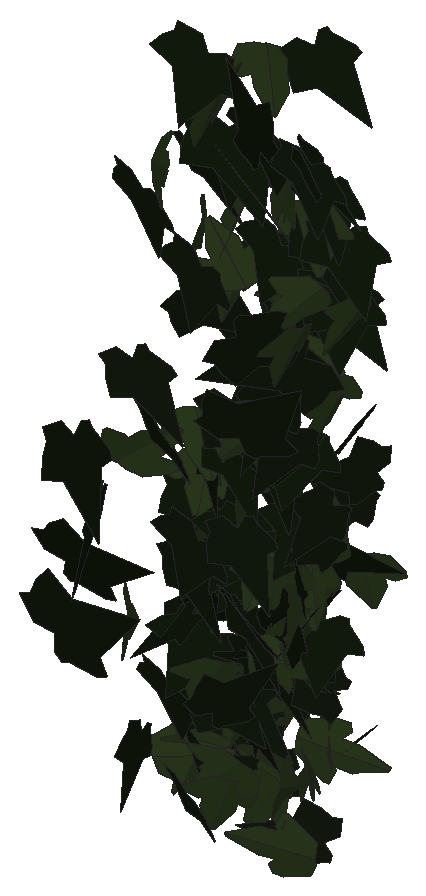
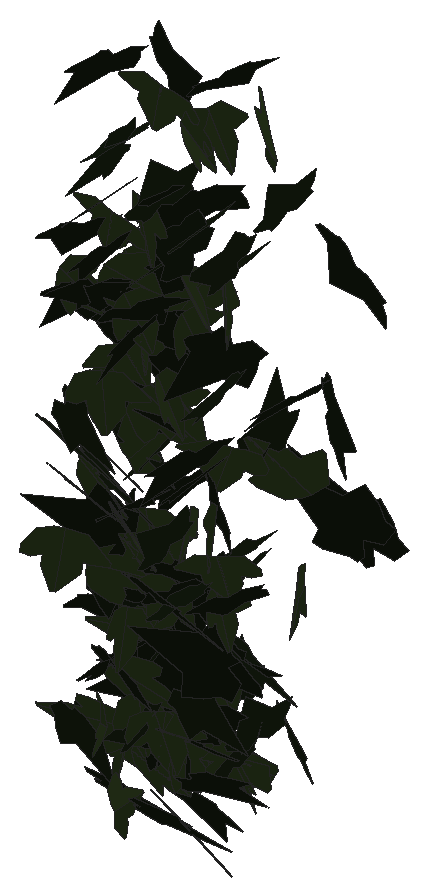
# SketchUp Ruby script. Lengths in inches.
U = 1.inch
M = Sketchup.active_model
def pt(a) = Geom::Point3d.new(a.map { |v| v * U })
def face(e, loops, mat)
  f = e.add_face(loops[0].map { |a| pt(a) })
  loops[1..].each { |l| e.add_face(l.map { |a| pt(a) }).erase! }
  f.material = f.back_material = mat if mat
  f
end
# faces: each face lists its corners as indices into pts; further lists are holes
def faces(e, pts, list, mat = nil) = list.each { |f| face(e, (f[0].is_a?(Array) ? f : [f]).map { |l| l.map { |i| pts[i] } }, mat) }
# xy, xz, yz: faces in a plane at the given z, y or x. An outline is a flat list of corners, or four numbers for a rectangle; further outlines are holes
def ring(l) = l.size == 4 ? [[l[0], l[1]], [l[2], l[1]], [l[2], l[3]], [l[0], l[3]]] : l.each_slice(2).to_a
def flat(e, list, mat, &to3) = list.each { |f| face(e, (f[0].is_a?(Array) ? f : [f]).map { |l| ring(l).map { |u, v| to3.(u, v) } }, mat) }
def xy(e, z, list, mat = nil) = flat(e, list, mat) { |x, y| [x, y, z] }
def xz(e, y, list, mat = nil) = flat(e, list, mat) { |x, z| [x, y, z] }
def yz(e, x, list, mat = nil) = flat(e, list, mat) { |y, z| [x, y, z] }
def lines(e, pts, list) = list.each { |a, b| e.add_line(pt(pts[a]), pt(pts[b])) }
# prism: a flat outline (further loops are holes) pulled along v
def prism(e, loops, v, mat = nil)
  f = face(e, loops, mat); d = Geom::Vector3d.new(v.map { |x| x * U })
  f.pushpull(f.normal.samedirection?(d) ? d.length : -d.length)
end
def box(e, o, s, mat = nil) = prism(e, [[o, [o[0] + s[0], o[1], o[2]], [o[0] + s[0], o[1] + s[1], o[2]], [o[0], o[1] + s[1], o[2]]]], [0, 0, s[2]], mat)
def at(x, y, z, deg = 0) = Geom::Transformation.translation(pt([x, y, z])) * Geom::Transformation.rotation(ORIGIN, Z_AXIS, deg.degrees)
def axes(o, x, y, z) = Geom::Transformation.new([*x, 0, *y, 0, *z, 0, *pt(o).to_a, 1])
def part(name) = M.definitions.add(name)
# library, detail: a bought-in or finely detailed component or shape, given as its bounding box
def library(name, o, s) = part(name).tap { |d| box(d.entities, o, s) }
def detail(e, o, s) = box(e.add_group.entities, o, s)
def put(e, d, t, mat = nil) = e.add_instance(d, t).tap { |i| i.material = mat if mat }
def group(e, t, mat = nil) = e.add_group.tap { |g| g.transformation = t; g.material = mat if mat }.entities
root = M.entities
M.materials.add("1026 AP 7946 SUNNY SIDE UP").color = [254, 231, 186]
M.materials.add("efeu1").color = [18, 25, 13]
M.materials.add("efeu2").color = [43, 57, 29]
c1 = part("ivyleaf_9")
p = [[1.54,2.16,1.25],[1.36,2.04,1.19],[-0.21,0.99,0.68],[-0.71,1.11,0.82],[-0.85,0.86,0.67],[-0.8,0.17,0.21],
  [-0.9,-0.01,0.1],[-0.67,-0.16,-0.02],[-0.08,-0.08,-0.05],[-0.03,-0.6,-0.4],[0.65,-0.88,-0.66],[0.83,-0.6,-0.49],
  [1.29,-0.42,-0.43],[1.8125,-0.07,-0.26],[1.21,0.44,0.15]]
faces(c1.entities,p,[[0,1,2,3,4,5,6,7,8,9,10,11,12,13,14]],"efeu1")
c2 = part("ivyleaf_10")
p = [[0,0.5,-0.03],[-0.0625,2.02,-0.43],[-0.19,2.01,-0.46],[-0.54,1.05,-0.29],[-0.52,0.625,-0.18],[-0.83,0.76,-0.28],
  [-1.16,0.64,-0.33],[-1.15,0.33,-0.24],[-0.77,-0.39,0.02],[-0.3,-0.51,0.16],[0.04,-0.48,0.23],[-0.02,2.01,-0.4375],
  [-0.06,2.01,-0.43],[0.04,-0.49,0.23],[0.67,-0.49,0.14],[1.38,0.36,-0.2],[1.375,0.51,-0.24],[0.81,0.65,-0.19],
  [0.62,0.59,-0.15],[0.6,1.09,-0.28],[0.5,1.23,-0.31]]
faces(c2.entities,p,[[0,1,2,3,4,5,6,7,8,9,10],[11,12,0,13,14,15,16,17,18,19,20]],"efeu2")
put(root,c1,axes([128.98,212.18,288.85],[0.31029,-0.29326,0.02774],[0.02209,-0.02501,-0.36428],[0.46278,0.19782,-0.00121]),"1026 AP 7946 SUNNY SIDE UP")
put(root,c2,axes([129.09,210.67,284.76],[-0.31965,-0.18826,0.23279],[0.23188,0.17392,0.28561],[-0.40163,0.25025,-0.02038]),"1026 AP 7946 SUNNY SIDE UP")
put(root,c1,axes([129.04,210.82,286.14],[0.1394,-0.3386,-0.12751],[0.0207,0.12846,-0.35713],[0.56545,0.07877,0.04451]),"1026 AP 7946 SUNNY SIDE UP")
put(root,c1,axes([129.14,212.12,283.58],[-0.05305,-0.33119,-0.07714],[0.03232,0.07122,-0.34228],[0.53228,-0.03734,0.0131]),"1026 AP 7946 SUNNY SIDE UP")
put(root,c2,axes([129.27,212.125,284.0625],[0.45145,0.17881,-0.05168],[-0.04942,-0.04614,-0.34796],[-0.28825,0.28796,-0.02128]),"1026 AP 7946 SUNNY SIDE UP")
put(root,c1,axes([128.88,209.61,283.53],[0.07526,-0.04022,0.3979],[0.48083,-0.23633,-0.06574],[0.37693,0.3095,0.00441]),"1026 AP 7946 SUNNY SIDE UP")
put(root,c2,axes([129.44,211.78,288.09],[0.15161,-0.31162,-0.1802],[-0.01395,0.17722,-0.33263],[0.56039,0.08872,0.04047]),"1026 AP 7946 SUNNY SIDE UP")
put(root,c1,axes([129.16,212.22,286.77],[0.23192,-0.3104,-0.0389],[-0.03271,0.02997,-0.35381],[0.49025,0.14884,-0.0052]),"1026 AP 7946 SUNNY SIDE UP")
put(root,c1,axes([129.63,211.27,282.24],[-0.41649,0.14606,-0.1242],[0.11868,-0.1102,-0.30691],[-0.27403,-0.26972,0.05584]),"1026 AP 7946 SUNNY SIDE UP")
put(root,c2,axes([129.53,211.8,283.26],[-0.04126,-0.32542,-0.02046],[-0.0011,0.01813,-0.33622],[0.51247,-0.02616,-0.00237]),"1026 AP 7946 SUNNY SIDE UP")
put(root,c2,axes([129.63,211.86,284.52],[-0.14659,0.22989,0.23773],[-0.24344,0.17841,-0.2479],[-0.44899,-0.17179,0.05679]),"1026 AP 7946 SUNNY SIDE UP")
put(root,c1,axes([129.25,210.73,288.93],[0.05276,-0.30959,0.21871],[0.07883,-0.20932,-0.32119],[0.58655,0.05598,0.02349]),"1026 AP 7946 SUNNY SIDE UP")
put(root,c2,axes([129.57,210,282.73],[0.14073,-0.21398,-0.33372],[-0.02347,0.32908,-0.22712],[0.60841,0.06219,0.06843]),"1026 AP 7946 SUNNY SIDE UP")
put(root,c1,axes([129.75,212.03,280.51],[-0.44826,-0.1148,0.09985],[-0.12089,-0.06874,-0.31513],[0.20373,-0.29337,0.0327]),"1026 AP 7946 SUNNY SIDE UP")
put(root,c1,axes([129.45,210.42,280.66],[-0.29729,0.01639,-0.31],[0.43122,-0.13818,-0.18602],[-0.19681,-0.32751,0.0607]),"1026 AP 7946 SUNNY SIDE UP")
put(root,c1,axes([129.34,211.22,281],[-0.02633,-0.26581,0.24746],[0.1188,-0.23918,-0.26696],[0.5523,0.03878,0.06922]),"1026 AP 7946 SUNNY SIDE UP")
put(root,c1,axes([129.56,211.5625,287.07],[-0.00988,-0.08955,-0.36536],[-0.03579,0.3536,-0.08963],[0.57326,0.02053,-0.01189]),"1026 AP 7946 SUNNY SIDE UP")
put(root,c1,axes([129.48,210.8,285.26],[0.40755,-0.2427,-0.19779],[0.25328,-0.10593,0.36397],[-0.4139,-0.3038,0.02797]),"1026 AP 7946 SUNNY SIDE UP")
put(root,c1,axes([129.57,212.22,289.14],[-0.01928,-0.32385,0.14098],[0.0022,-0.13882,-0.33462],[0.55394,-0.01072,0.00623]),"1026 AP 7946 SUNNY SIDE UP")
put(root,c1,axes([129.31,208.84,282.92],[-0.04634,0.08615,0.46305],[0.4592,-0.34261,0.08547],[0.55308,0.29167,-0.03217]),"1026 AP 7946 SUNNY SIDE UP")
put(root,c1,axes([129.93,211.96,281.73],[-0.25677,0.20577,-0.20613],[0.09457,-0.20189,-0.2641],[-0.44259,-0.16252,0.06316]),"1026 AP 7946 SUNNY SIDE UP")
put(root,c2,axes([129.77,212.13,288.15],[0.27324,-0.30063,0.10989],[0.05657,-0.10417,-0.35774],[0.4993,0.17632,-0.0196]),"1026 AP 7946 SUNNY SIDE UP")
put(root,c1,axes([129.59,211.45,280.53],[0.01277,-0.26341,0.28842],[0.03471,-0.28075,-0.27297],[0.60516,0.02166,0.00957]),"1026 AP 7946 SUNNY SIDE UP")
put(root,c1,axes([129.6,211.74,284.6875],[-0.15114,-0.00468,-0.3375],[0.49212,-0.10221,-0.0937],[-0.15225,-0.32573,0.03216]),"1026 AP 7946 SUNNY SIDE UP")
put(root,c1,axes([129.89,211.37,281.95],[-0.42373,-0.2031,-0.00622],[0.02623,-0.01404,-0.34702],[0.31836,-0.26916,0.02032]),"1026 AP 7946 SUNNY SIDE UP")
put(root,c1,axes([129.74,209.17,284.96],[-0.30278,0.08323,-0.42338],[0.5409,-0.22815,-0.21473],[-0.3783,-0.39283,0.03184]),"1026 AP 7946 SUNNY SIDE UP")
put(root,c2,axes([129.89,211,280.27],[0.32015,-0.2617,-0.01845],[-0.03294,0.00449,-0.34127],[0.41099,0.20422,-0.01298]),"1026 AP 7946 SUNNY SIDE UP")
put(root,c1,axes([130.23,211.95,279.81],[-0.2866,0.22726,0.15585],[-0.16229,0.10936,-0.29927],[-0.3962,-0.20919,0.00986]),"1026 AP 7946 SUNNY SIDE UP")
put(root,c2,axes([129.9,211.96,290.4375],[0.15864,-0.30207,0.16275],[0.04643,-0.15818,-0.32838],[0.53525,0.10325,-0.01975]),"1026 AP 7946 SUNNY SIDE UP")
put(root,c1,axes([129.57,211.67,282.18],[0.24071,0.27262,-0.17899],[0.09189,0.16746,0.32187],[0.50129,-0.16161,0.02694]),"1026 AP 7946 SUNNY SIDE UP")
put(root,c2,axes([129.97,211.35,290.31],[-0.01407,-0.35184,0.06304],[0.00713,-0.06332,-0.3629],[0.56205,-0.00801,0.00618]),"1026 AP 7946 SUNNY SIDE UP")
put(root,c2,axes([129.74,211.32,285.24],[0.474,0.18788,0.07671],[0.12034,0.01557,-0.3648],[-0.29344,0.30986,-0.0257]),"1026 AP 7946 SUNNY SIDE UP")
put(root,c2,axes([129.78,211.0625,280.4],[-0.36542,-0.13235,-0.18939],[0.27678,0.05857,-0.27345],[0.22267,-0.29,0.02909]),"1026 AP 7946 SUNNY SIDE UP")
put(root,c1,axes([129.78,212.4,283.36],[-0.07065,-0.29446,0.19494],[0.05816,-0.19536,-0.30261],[0.54872,-0.01721,0.05718]),"1026 AP 7946 SUNNY SIDE UP")
put(root,c1,axes([129.91,211.3,291],[-0.21379,-0.33817,0.12317],[-0.04298,-0.11978,-0.37571],[0.56338,-0.13747,0.01808]),"1026 AP 7946 SUNNY SIDE UP")
put(root,c1,axes([129.73,211.01,283.26],[0.20783,-0.33524,-0.04471],[-0.04431,0.03347,-0.37076],[0.5293,0.13444,-0.01348]),"1026 AP 7946 SUNNY SIDE UP")
put(root,c2,axes([129.6,210.89,280.2],[0.19503,-0.05407,-0.30723],[0.46486,0.09119,0.11028],[0.10288,-0.30956,0.08413]),"1026 AP 7946 SUNNY SIDE UP")
put(root,c2,axes([129.74,210.48,289.64],[0.08213,-0.17038,-0.37165],[0.19188,-0.33856,0.18143],[-0.59583,-0.13251,0.0072]),"1026 AP 7946 SUNNY SIDE UP")
put(root,c1,axes([129.86,211.16,283.5],[-0.14287,-0.28812,0.20162],[0.01636,-0.20606,-0.3062],[0.54888,-0.06886,0.06161]),"1026 AP 7946 SUNNY SIDE UP")
put(root,c2,axes([129.98,211.9,287.41],[-0.07131,-0.31594,0.14114],[0.07394,-0.14434,-0.3235],[0.53755,-0.02206,0.06322]),"1026 AP 7946 SUNNY SIDE UP")
put(root,c1,axes([129.83,211.93,289.51],[-0.13347,-0.34189,-0.20315],[0.09331,0.18635,-0.36164],[0.61201,-0.10297,0.01083]),"1026 AP 7946 SUNNY SIDE UP")
put(root,c1,axes([130.09,211.68,279.98],[-0.45971,-0.04195,-0.13367],[0.20684,-0.00801,-0.30328],[0.05515,-0.31966,0.02323]),"1026 AP 7946 SUNNY SIDE UP")
put(root,c2,axes([130.16,211.625,287.58],[0.20429,0.34869,0.07074],[-0.08425,-0.05094,0.38163],[0.55182,-0.13687,0.03208]),"1026 AP 7946 SUNNY SIDE UP")
put(root,c2,axes([130.07,211.93,280.66],[-0.06327,-0.26305,0.17177],[0.06523,-0.17262,-0.26886],[0.48662,-0.01106,0.05837]),"1026 AP 7946 SUNNY SIDE UP")
put(root,c1,axes([129.74,212.18,288.74],[0.25367,-0.2557,0.21436],[0.16216,-0.18259,-0.31242],[0.49387,0.19129,-0.00752]),"1026 AP 7946 SUNNY SIDE UP")
put(root,c1,axes([129.98,211.07,287.83],[-0.07442,-0.31588,0.19649],[0.0005,-0.19413,-0.32918],[0.58167,-0.04025,0.02542]),"1026 AP 7946 SUNNY SIDE UP")
put(root,c1,axes([130.44,211.88,280.92],[-0.4647,0.03392,0.10972],[-0.17546,-0.09083,-0.29026],[0.00058,-0.30065,0.09812]),"1026 AP 7946 SUNNY SIDE UP")
put(root,c2,axes([130.26,211.1,281.66],[-0.27905,-0.2664,0.10917],[-0.07268,-0.09821,-0.32997],[0.44581,-0.18276,0.01454]),"1026 AP 7946 SUNNY SIDE UP")
put(root,c2,axes([130.35,212.12,281.19],[-0.42749,-0.14965,0.09816],[-0.11783,-0.06288,-0.31953],[0.25364,-0.28143,0.01701]),"1026 AP 7946 SUNNY SIDE UP")
put(root,c1,axes([129.97,211.82,285.37],[0.11708,-0.3568,-0.21301],[-0.03229,0.20459,-0.37379],[0.64603,0.07489,0.01992]),"1026 AP 7946 SUNNY SIDE UP")
put(root,c2,axes([130.25,212.08,286.4],[0.08507,-0.34302,0.04229],[0.0026,-0.04327,-0.35796],[0.54358,0.05389,-0.00491]),"1026 AP 7946 SUNNY SIDE UP")
put(root,c2,axes([130.21,211.57,284.16],[0.21798,-0.21477,-0.21885],[0.04701,0.24117,-0.23101],[0.47131,0.07528,0.12426]),"1026 AP 7946 SUNNY SIDE UP")
put(root,c2,axes([130.33,211.98,280.93],[-0.07069,0.29943,-0.20892],[-0.03244,0.20361,0.313],[0.56922,0.04879,-0.00811]),"1026 AP 7946 SUNNY SIDE UP")
put(root,c1,axes([130.33,211.79,283.52],[-0.43734,-0.19791,-0.00507],[0.02987,-0.02017,-0.35065],[0.30982,-0.27743,0.02665]),"1026 AP 7946 SUNNY SIDE UP")
put(root,c1,axes([130.59,212.15,283.27],[-0.53377,0.11963,0.02066],[-0.04705,-0.02689,-0.36916],[-0.18466,-0.33895,0.03434]),"1026 AP 7946 SUNNY SIDE UP")
put(root,c1,axes([130.32,211.85,283.16],[-0.28947,-0.2616,0.07292],[-0.05448,-0.06395,-0.32981],[0.42326,-0.18714,0.00742]),"1026 AP 7946 SUNNY SIDE UP")
put(root,c1,axes([130.65,212.01,279.74],[-0.43261,0.08348,0.13003],[-0.21368,-0.02327,-0.29054],[-0.10325,-0.3016,0.0565]),"1026 AP 7946 SUNNY SIDE UP")
put(root,c1,axes([130.1,211.6,284.86],[0.08809,-0.35626,-0.02097],[-0.0143,0.01713,-0.37137],[0.56074,0.05641,-0.00618]),"1026 AP 7946 SUNNY SIDE UP")
put(root,c1,axes([130.03,212.29,284.18],[0.15924,-0.30773,0.14662],[0.07574,-0.13581,-0.33453],[0.52888,0.11211,0.00376]),"1026 AP 7946 SUNNY SIDE UP")
put(root,c1,axes([130.27,211.86,281],[-0.13516,-0.28439,-0.17093],[0.08103,0.15605,-0.30513],[0.51004,-0.10016,0.00318]),"1026 AP 7946 SUNNY SIDE UP")
put(root,c1,axes([130.17,212.26,289.41],[-0.03595,-0.30299,0.27858],[0.12253,-0.27078,-0.30543],[0.62855,0.03546,0.07548]),"1026 AP 7946 SUNNY SIDE UP")
put(root,c1,axes([130.19,211.33,281.2],[-0.0263,-0.18766,-0.30519],[0.26953,0.2532,-0.17436],[0.47942,-0.15264,0.08128]),"1026 AP 7946 SUNNY SIDE UP")
put(root,c1,axes([130.15,211.41,282.52],[0.25666,-0.18081,0.22477],[0.18419,-0.18751,-0.25029],[0.40708,0.19884,-0.02847]),"1026 AP 7946 SUNNY SIDE UP")
put(root,c1,axes([130.21,208.06,286.55],[-0.27026,-0.07851,-0.42642],[0.66177,-0.03067,-0.17441],[0.00206,-0.44673,0.08421]),"1026 AP 7946 SUNNY SIDE UP")
put(root,c2,axes([130.5,211.66,282.97],[-0.47387,0.10493,-0.0785],[0.10243,-0.04593,-0.32828],[-0.17695,-0.30759,0.0202]),"1026 AP 7946 SUNNY SIDE UP")
put(root,c1,axes([130.22,211.74,280.77],[0.1249,-0.0816,-0.36921],[0.55808,-0.0765,0.09866],[-0.1475,-0.35856,0.06067]),"1026 AP 7946 SUNNY SIDE UP")
put(root,c1,axes([130.59,212.34,287.66],[-0.27499,-0.30562,0.06225],[-0.02113,-0.06382,-0.36255],[0.48994,-0.17429,0.0193]),"1026 AP 7946 SUNNY SIDE UP")
put(root,c2,axes([130.42,211.94,290.86],[0.54317,-0.00947,0.1118],[0.17042,-0.00835,-0.35601],[0.01813,0.36201,-0.00317]),"1026 AP 7946 SUNNY SIDE UP")
put(root,c2,axes([130.875,210.65,280.55],[-0.41934,-0.04506,0.1981],[-0.27105,-0.10543,-0.272],[0.15237,-0.31158,0.06132]),"1026 AP 7946 SUNNY SIDE UP")
put(root,c2,axes([131.03,211.51,280.16],[0.03821,-0.06202,-0.35009],[-0.42407,0.20891,-0.05798],[0.33854,0.26869,-0.03312]),"1026 AP 7946 SUNNY SIDE UP")
put(root,c2,axes([131.02,211.95,281.68],[0.20781,-0.02697,-0.31376],[-0.46841,0.06264,-0.13859],[0.10723,0.32589,0.00267]),"1026 AP 7946 SUNNY SIDE UP")
put(root,c2,axes([130.93,211.43,285.66],[-0.27437,-0.2565,0.2591],[-0.19265,-0.22207,-0.32034],[0.53271,-0.21242,0.0176]),"1026 AP 7946 SUNNY SIDE UP")
put(root,c2,axes([130.82,210.64,280.21],[-0.34326,-0.23742,0.07887],[-0.05126,-0.07551,-0.3316],[0.38955,-0.21915,0.02587]),"1026 AP 7946 SUNNY SIDE UP")
put(root,c2,axes([130.74,211.93,288.94],[0.38784,-0.22497,-0.11929],[-0.04237,0.13573,-0.33369],[0.39466,0.23565,0.0814]),"1026 AP 7946 SUNNY SIDE UP")
put(root,c1,axes([130.64,211.97,288],[-0.12196,-0.29183,0.19282],[-0.02555,-0.19021,-0.31084],[0.54595,-0.07409,0.02852]),"1026 AP 7946 SUNNY SIDE UP")
put(root,c1,axes([130.41,211.36,281.86],[0.1263,0.00693,-0.32666],[0.27861,0.27036,0.0539],[0.4137,-0.18419,0.06343]),"1026 AP 7946 SUNNY SIDE UP")
put(root,c2,axes([130.84,211.88,281.1875],[-0.25378,-0.28316,0.00827],[0.01653,-0.01707,-0.33538],[0.44519,-0.16078,0.01717]),"1026 AP 7946 SUNNY SIDE UP")
put(root,c1,axes([130.55,212.14,281.18],[0.27127,-0.28105,0.01707],[-0.00698,-0.02401,-0.33946],[0.44279,0.1718,-0.01581]),"1026 AP 7946 SUNNY SIDE UP")
put(root,c1,axes([130.46,211.5,281.57],[0.37132,0.08955,0.22023],[0.33491,0.03466,-0.25776],[-0.14183,0.3163,-0.03209]),"1026 AP 7946 SUNNY SIDE UP")
put(root,c2,axes([130.87,212.03,287.43],[-0.13479,-0.32378,0.11475],[0.01275,-0.11859,-0.34373],[0.5392,-0.07814,0.03682]),"1026 AP 7946 SUNNY SIDE UP")
put(root,c1,axes([130.59,211.34,282.55],[0.17324,-0.33325,0.0462],[0.00667,-0.0478,-0.36169],[0.52909,0.10972,-0.01057]),"1026 AP 7946 SUNNY SIDE UP")
put(root,c1,axes([130.7,212.07,287.16],[0.19216,-0.28818,-0.19931],[-0.13759,0.17112,-0.32124],[0.52667,0.14985,-0.0112]),"1026 AP 7946 SUNNY SIDE UP")
put(root,c2,axes([130.875,212.33,279.83],[-0.11175,0.05265,-0.32907],[-0.06392,-0.32619,-0.04793],[-0.50548,0.02961,0.07881]),"1026 AP 7946 SUNNY SIDE UP")
put(root,c2,axes([130.92,212.0625,282.58],[-0.09734,-0.30946,-0.12062],[0.08296,0.10656,-0.32312],[0.51261,-0.07601,0.02939]),"1026 AP 7946 SUNNY SIDE UP")
put(root,c2,axes([130.92,211.3125,283.51],[0.29384,0.25441,-0.14933],[-0.10083,-0.13398,-0.32495],[-0.45039,0.19597,-0.02468]),"1026 AP 7946 SUNNY SIDE UP")
put(root,c2,axes([131.09,211.66,284.99],[-0.13959,-0.11042,-0.344],[-0.20257,-0.30956,0.1392],[-0.51357,0.15211,0.0386]),"1026 AP 7946 SUNNY SIDE UP")
put(root,c1,axes([131.27,210.72,290.32],[0.00792,-0.00458,0.42375],[-0.16731,0.39738,0.00822],[-0.62485,-0.10646,0.00317]),"1026 AP 7946 SUNNY SIDE UP")
put(root,c1,axes([130.78,209.8,280.47],[0.34127,-0.18212,-0.18513],[0.23814,-0.09681,0.29061],[-0.32283,-0.26393,0.01866]),"1026 AP 7946 SUNNY SIDE UP")
put(root,c2,axes([131.13,211.56,287.06],[0.12315,-0.32267,-0.18992],[-0.06581,0.17766,-0.34102],[0.57918,0.08879,0.00163]),"1026 AP 7946 SUNNY SIDE UP")
put(root,c2,axes([130.8,211.86,283.52],[0.29843,-0.22859,-0.18702],[0.25267,-0.09714,0.30067],[-0.38166,-0.24304,0.05282]),"1026 AP 7946 SUNNY SIDE UP")
put(root,c1,axes([130.92,210.73,284.2],[0.06829,-0.34078,-0.123],[-0.046,0.11459,-0.35296],[0.56491,0.05052,-0.01387]),"1026 AP 7946 SUNNY SIDE UP")
put(root,c1,axes([130.91,211.54,284.91],[0.07036,-0.31204,0.11333],[0.00694,-0.11222,-0.32521],[0.52113,0.04362,-0.01097]),"1026 AP 7946 SUNNY SIDE UP")
put(root,c2,axes([131.12,211.87,286.63],[0.34976,0.24975,-0.14014],[-0.13255,-0.10892,-0.34506],[-0.42821,0.23771,-0.00765]),"1026 AP 7946 SUNNY SIDE UP")
put(root,c1,axes([130.88,211.35,281.99],[0.31958,-0.29615,-0.06152],[-0.07751,0.03645,-0.36926],[0.46815,0.2082,-0.01914]),"1026 AP 7946 SUNNY SIDE UP")
put(root,c1,axes([131.18,211.31,286.18],[-0.52141,0.05376,-0.24378],[0.35468,-0.08085,-0.34458],[-0.14196,-0.39945,0.03446]),"1026 AP 7946 SUNNY SIDE UP")
put(root,c1,axes([131.55,211.3,286.86],[0.00731,-0.04482,-0.41684],[-0.38535,-0.3231,0.0321],[-0.51064,0.24319,-0.03019]),"1026 AP 7946 SUNNY SIDE UP")
put(root,c1,axes([130.98,210.69,287.26],[0.04697,0.02241,-0.41924],[-0.0406,0.40745,0.02354],[0.63977,0.02421,0.03227]),"1026 AP 7946 SUNNY SIDE UP")
put(root,c2,axes([131.31,211.15,283.58],[-0.43655,-0.17235,0.06034],[-0.05159,-0.05949,-0.33531],[0.28205,-0.27765,0.03206]),"1026 AP 7946 SUNNY SIDE UP")
put(root,c1,axes([131.125,212.05,281.78],[-0.35791,-0.01626,-0.24221],[0.36982,-0.03437,-0.23242],[-0.02119,-0.32536,0.03473]),"1026 AP 7946 SUNNY SIDE UP")
put(root,c2,axes([131.42,211.89,283.13],[-0.08203,-0.10298,0.36152],[-0.19561,-0.32897,-0.12023],[0.54171,-0.13438,0.01133]),"1026 AP 7946 SUNNY SIDE UP")
put(root,c2,axes([131.34,212.09,286.1],[-0.4154,-0.20689,0.02255],[-0.00541,-0.03292,-0.34501],[0.32729,-0.26313,0.02292]),"1026 AP 7946 SUNNY SIDE UP")
put(root,c2,axes([131.32,211.72,280.36],[-0.27957,0.24998,0.07178],[-0.10418,0.03618,-0.31406],[-0.39391,-0.18698,0.03211]),"1026 AP 7946 SUNNY SIDE UP")
put(root,c1,axes([131.61,211,283],[0.05018,-0.00341,-0.39736],[-0.60213,0.04602,-0.03279],[0.07256,0.38426,0.00269]),"1026 AP 7946 SUNNY SIDE UP")
put(root,c2,axes([131.39,211.68,287.62],[-0.1778,-0.18362,0.29394],[-0.05668,-0.29361,-0.21033],[0.53189,-0.09267,0.07584]),"1026 AP 7946 SUNNY SIDE UP")
put(root,c2,axes([131.39,210.85,280.28],[0.39897,-0.17888,-0.11336],[-0.14116,0.06186,-0.31946],[0.29761,0.26915,0.00044]),"1026 AP 7946 SUNNY SIDE UP")
put(root,c1,axes([131.55,211.33,285.3],[-0.26539,0.29581,-0.07573],[0.03539,-0.07363,-0.35087],[-0.47861,-0.16947,0.01605]),"1026 AP 7946 SUNNY SIDE UP")
put(root,c1,axes([131.32,211.57,285.43],[-0.40042,-0.19102,-0.11293],[0.1678,0.03769,-0.32606],[0.30196,-0.27424,0.03144]),"1026 AP 7946 SUNNY SIDE UP")
put(root,c1,axes([131.16,212.21,288.34],[0.07037,-0.35414,-0.08488],[-0.0397,0.07776,-0.36696],[0.56964,0.04917,-0.01509]),"1026 AP 7946 SUNNY SIDE UP")
put(root,c1,axes([131.09,210.57,285.83],[-0.23985,-0.01488,0.3415],[0.50509,-0.09849,0.14711],[0.1314,0.35144,0.05791]),"1026 AP 7946 SUNNY SIDE UP")
put(root,c1,axes([131.34,211.6875,283.98],[-0.2146,-0.25887,0.16155],[-0.05548,-0.15884,-0.29989],[0.47387,-0.13583,0.03805]),"1026 AP 7946 SUNNY SIDE UP")
put(root,c1,axes([131.58,211.9,281.49],[-0.15593,-0.35647,0.01444],[0.01081,0.01474,0.38125],[-0.56097,0.09937,0.00333]),"1026 AP 7946 SUNNY SIDE UP")
put(root,c2,axes([131,211.25,282.01],[0.04148,-0.01659,-0.36568],[0.52178,0.1282,0.01999],[0.19945,-0.33195,0.02376]),"1026 AP 7946 SUNNY SIDE UP")
put(root,c1,axes([131.2,212.08,291.21],[0.10607,-0.28841,-0.23488],[-0.01371,0.22883,-0.3017],[0.57632,0.05853,0.03605]),"1026 AP 7946 SUNNY SIDE UP")
put(root,c1,axes([131.22,209.85,281.92],[-0.05227,-0.03335,0.3425],[0.45509,0.16446,0.04774],[-0.26313,0.29106,0.01453]),"1026 AP 7946 SUNNY SIDE UP")
put(root,c1,axes([131.24,212.29,289.03],[0.0032,-0.36094,0.06924],[0.00619,-0.06923,-0.37223],[0.57787,0.00274,0.0036]),"1026 AP 7946 SUNNY SIDE UP")
put(root,c2,axes([131.22,211.99,288.66],[0.53841,-0.03995,0.13733],[0.20107,-0.05084,-0.35378],[0.08718,0.36399,-0.03215]),"1026 AP 7946 SUNNY SIDE UP")
put(root,c1,axes([131.84,211.36,279.44],[-0.34546,0.14514,0.18021],[-0.28822,0.02888,-0.26291],[-0.20967,-0.27883,0.06449]),"1026 AP 7946 SUNNY SIDE UP")
put(root,c1,axes([131.52,211.19,285.78],[-0.5109,-0.01231,-0.15509],[0.23725,-0.03929,-0.33255],[-0.00851,-0.35591,0.03996]),"1026 AP 7946 SUNNY SIDE UP")
put(root,c1,axes([131.25,211.77,289.69],[0.38648,-0.23369,-0.15401],[-0.14853,0.11542,-0.34827],[0.40895,0.26277,0.01906]),"1026 AP 7946 SUNNY SIDE UP")
put(root,c2,axes([131.55,211.43,282.79],[-0.09239,-0.38326,0.07652],[-0.00019,-0.07729,-0.39973],[0.61452,-0.05764,0.01138]),"1026 AP 7946 SUNNY SIDE UP")
put(root,c2,axes([131.37,212.06,280.82],[-0.08254,0.15862,-0.28692],[0.13624,-0.26564,-0.17368],[-0.4865,-0.1013,0.00004]),"1026 AP 7946 SUNNY SIDE UP")
put(root,c2,axes([131.57,211.92,285.88],[0.04258,-0.30745,0.1838],[0.04675,-0.1781,-0.31876],[0.55837,0.03836,0.01267]),"1026 AP 7946 SUNNY SIDE UP")
put(root,c1,axes([131.67,211.06,283.7],[0.17672,-0.03809,-0.32079],[-0.4143,0.16764,-0.1182],[0.26709,0.28523,0.02891]),"1026 AP 7946 SUNNY SIDE UP")
put(root,c1,axes([131.67,211.72,282.95],[-0.25979,0.11675,-0.27306],[0.22543,-0.23302,-0.19868],[-0.39681,-0.20882,0.0659]),"1026 AP 7946 SUNNY SIDE UP")
put(root,c1,axes([131.41,211.68,289.62],[-0.03668,-0.33618,0.11643],[0.05718,-0.11683,-0.34514],[0.55571,-0.01016,0.0432]),"1026 AP 7946 SUNNY SIDE UP")
put(root,c2,axes([131.66,211.01,287.36],[-0.03115,-0.37311,0.07326],[0.00707,-0.07356,-0.38525],[0.59782,-0.01857,0.00838]),"1026 AP 7946 SUNNY SIDE UP")
put(root,c1,axes([131.55,212.11,287.53],[-0.26221,-0.30477,-0.10121],[0.11308,0.0703,-0.3563],[0.48978,-0.17939,0.02808]),"1026 AP 7946 SUNNY SIDE UP")
put(root,c1,axes([131.58,211.73,282.58],[-0.23324,-0.29881,-0.04217],[0.05808,0.02538,-0.3428],[0.47031,-0.15132,0.02142]),"1026 AP 7946 SUNNY SIDE UP")
put(root,c2,axes([131.43,211.6,283.45],[0.4956,-0.09418,0.19757],[0.26686,-0.09883,-0.33698],[0.20534,0.35575,-0.03892]),"1026 AP 7946 SUNNY SIDE UP")
put(root,c2,axes([132.08,210.57,279.6875],[-0.00204,0.04377,0.36555],[-0.51222,-0.14576,0.01645],[0.23071,-0.32324,0.03977]),"1026 AP 7946 SUNNY SIDE UP")
put(root,c1,axes([131.8,212.2,284.48],[-0.4867,0.01475,-0.12273],[0.17458,-0.09067,-0.30906],[-0.07212,-0.31906,0.08013]),"1026 AP 7946 SUNNY SIDE UP")
put(root,c2,axes([132.07,211.5,284.23],[-0.11156,0.12848,0.31099],[-0.48887,0.07015,-0.10589],[-0.16137,-0.30133,0.10577]),"1026 AP 7946 SUNNY SIDE UP")
put(root,c2,axes([131.76,210.62,280.61],[0.01247,-0.15982,-0.30355],[0.0321,0.29351,-0.16223],[0.52484,-0.01416,0.01713]),"1026 AP 7946 SUNNY SIDE UP")
put(root,c1,axes([131.9375,211.93,280.72],[-0.17906,0.28632,-0.08231],[0.02803,-0.08057,-0.31764],[-0.46726,-0.11456,0.01249]),"1026 AP 7946 SUNNY SIDE UP")
put(root,c1,axes([131.53,212.0625,287.54],[0.04017,-0.28105,-0.2252],[0.05388,0.2185,-0.28609],[0.55571,-0.00087,0.04402]),"1026 AP 7946 SUNNY SIDE UP")
put(root,c1,axes([131.89,212.14,285.57],[-0.28981,0.22067,-0.20178],[0.18012,-0.16091,-0.29686],[-0.42898,-0.21664,0.01167]),"1026 AP 7946 SUNNY SIDE UP")
put(root,c2,axes([131.91,210.71,283.3],[0.21723,-0.31169,-0.22298],[-0.10019,0.20611,-0.34933],[0.5866,0.15063,0.02291]),"1026 AP 7946 SUNNY SIDE UP")
put(root,c1,axes([131.38,211.78,283.67],[0.24441,-0.02512,0.30597],[0.43035,-0.12104,-0.15874],[0.18619,0.31274,-0.03475]),"1026 AP 7946 SUNNY SIDE UP")
put(root,c1,axes([131.68,212.08,288.44],[-0.09413,-0.32824,-0.10654],[0.07081,0.0947,-0.34212],[0.5356,-0.07021,0.0265]),"1026 AP 7946 SUNNY SIDE UP")
put(root,c1,axes([131.96,211.43,284.64],[-0.46696,0.02847,-0.1557],[0.2209,-0.08436,-0.30092],[-0.09903,-0.32244,0.06295]),"1026 AP 7946 SUNNY SIDE UP")
put(root,c2,axes([131.45,211.77,280.66],[-0.0519,-0.06697,-0.37301],[0.57681,-0.03289,-0.0284],[-0.04284,-0.36171,0.06944]),"1026 AP 7946 SUNNY SIDE UP")
put(root,c1,axes([132.17,211.29,284.3],[-0.42173,0.20128,-0.03016],[0.01257,-0.03987,-0.34457],[-0.31984,-0.26696,0.02623]),"1026 AP 7946 SUNNY SIDE UP")
put(root,c1,axes([132.26,211.98,285.05],[-0.39523,0.21093,0.07273],[-0.1249,0.01247,-0.33537],[-0.32605,-0.26046,0.04031]),"1026 AP 7946 SUNNY SIDE UP")
put(root,c2,axes([131.97,211.97,287.48],[-0.01317,-0.28435,0.2058],[-0.00658,-0.20134,-0.29423],[0.54784,-0.00925,0.00142]),"1026 AP 7946 SUNNY SIDE UP")
put(root,c2,axes([131.97,212.15,283.47],[-0.46473,-0.18194,-0.03566],[0.07307,-0.01174,-0.35587],[0.28159,-0.29722,0.03349]),"1026 AP 7946 SUNNY SIDE UP")
